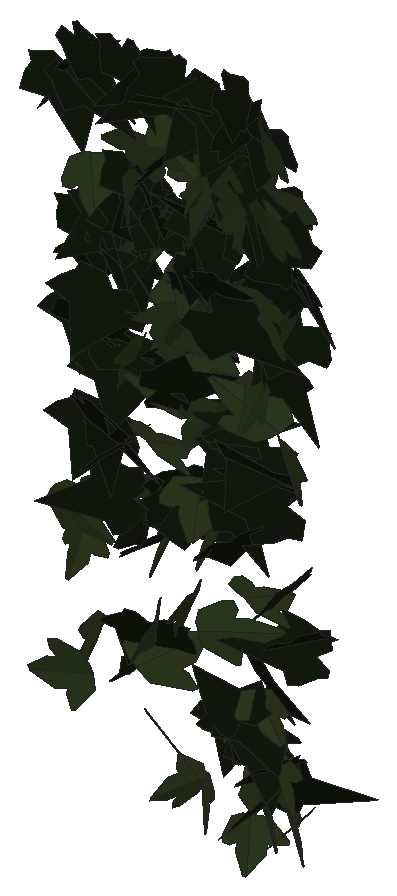
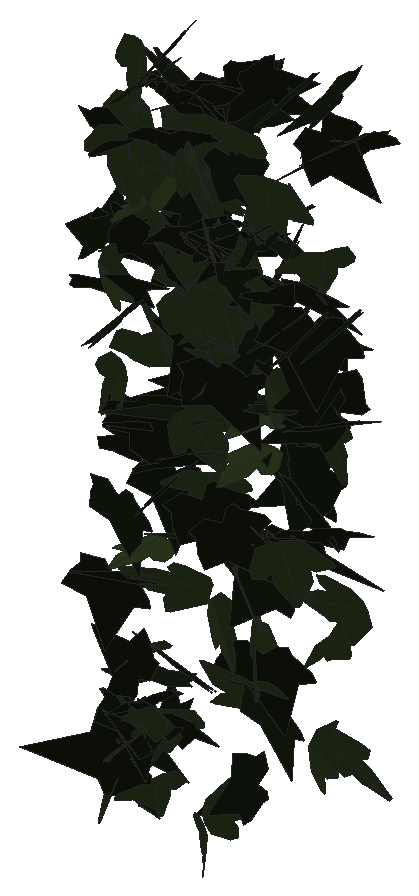
# SketchUp Ruby script. Lengths in inches.
U = 1.inch
M = Sketchup.active_model
def pt(a) = Geom::Point3d.new(a.map { |v| v * U })
def face(e, loops, mat)
  f = e.add_face(loops[0].map { |a| pt(a) })
  loops[1..].each { |l| e.add_face(l.map { |a| pt(a) }).erase! }
  f.material = f.back_material = mat if mat
  f
end
# faces: each face lists its corners as indices into pts; further lists are holes
def faces(e, pts, list, mat = nil) = list.each { |f| face(e, (f[0].is_a?(Array) ? f : [f]).map { |l| l.map { |i| pts[i] } }, mat) }
# xy, xz, yz: faces in a plane at the given z, y or x. An outline is a flat list of corners, or four numbers for a rectangle; further outlines are holes
def ring(l) = l.size == 4 ? [[l[0], l[1]], [l[2], l[1]], [l[2], l[3]], [l[0], l[3]]] : l.each_slice(2).to_a
def flat(e, list, mat, &to3) = list.each { |f| face(e, (f[0].is_a?(Array) ? f : [f]).map { |l| ring(l).map { |u, v| to3.(u, v) } }, mat) }
def xy(e, z, list, mat = nil) = flat(e, list, mat) { |x, y| [x, y, z] }
def xz(e, y, list, mat = nil) = flat(e, list, mat) { |x, z| [x, y, z] }
def yz(e, x, list, mat = nil) = flat(e, list, mat) { |y, z| [x, y, z] }
def lines(e, pts, list) = list.each { |a, b| e.add_line(pt(pts[a]), pt(pts[b])) }
# prism: a flat outline (further loops are holes) pulled along v
def prism(e, loops, v, mat = nil)
  f = face(e, loops, mat); d = Geom::Vector3d.new(v.map { |x| x * U })
  f.pushpull(f.normal.samedirection?(d) ? d.length : -d.length)
end
def box(e, o, s, mat = nil) = prism(e, [[o, [o[0] + s[0], o[1], o[2]], [o[0] + s[0], o[1] + s[1], o[2]], [o[0], o[1] + s[1], o[2]]]], [0, 0, s[2]], mat)
def at(x, y, z, deg = 0) = Geom::Transformation.translation(pt([x, y, z])) * Geom::Transformation.rotation(ORIGIN, Z_AXIS, deg.degrees)
def axes(o, x, y, z) = Geom::Transformation.new([*x, 0, *y, 0, *z, 0, *pt(o).to_a, 1])
def part(name) = M.definitions.add(name)
# library, detail: a bought-in or finely detailed component or shape, given as its bounding box
def library(name, o, s) = part(name).tap { |d| box(d.entities, o, s) }
def detail(e, o, s) = box(e.add_group.entities, o, s)
def put(e, d, t, mat = nil) = e.add_instance(d, t).tap { |i| i.material = mat if mat }
def group(e, t, mat = nil) = e.add_group.tap { |g| g.transformation = t; g.material = mat if mat }.entities
root = M.entities
M.materials.add("1026 AP 7946 SUNNY SIDE UP").color = [254, 231, 186]
M.materials.add("efeu1").color = [18, 25, 13]
M.materials.add("efeu2").color = [43, 57, 29]
c1 = part("ivyleaf_9")
p = [[1.54,2.16,1.25],[1.36,2.04,1.19],[-0.21,0.99,0.68],[-0.71,1.11,0.82],[-0.85,0.86,0.67],[-0.8,0.17,0.21],
  [-0.9,-0.01,0.1],[-0.67,-0.16,-0.02],[-0.08,-0.08,-0.05],[-0.03,-0.6,-0.4],[0.65,-0.88,-0.66],[0.83,-0.6,-0.49],
  [1.29,-0.42,-0.43],[1.8125,-0.07,-0.26],[1.21,0.44,0.15]]
faces(c1.entities,p,[[0,1,2,3,4,5,6,7,8,9,10,11,12,13,14]],"efeu1")
c2 = part("ivyleaf_10")
p = [[0,0.5,-0.03],[-0.0625,2.02,-0.43],[-0.19,2.01,-0.46],[-0.54,1.05,-0.29],[-0.52,0.625,-0.18],[-0.83,0.76,-0.28],
  [-1.16,0.64,-0.33],[-1.15,0.33,-0.24],[-0.77,-0.39,0.02],[-0.3,-0.51,0.16],[0.04,-0.48,0.23],[-0.02,2.01,-0.4375],
  [-0.06,2.01,-0.43],[0.04,-0.49,0.23],[0.67,-0.49,0.14],[1.38,0.36,-0.2],[1.375,0.51,-0.24],[0.81,0.65,-0.19],
  [0.62,0.59,-0.15],[0.6,1.09,-0.28],[0.5,1.23,-0.31]]
faces(c2.entities,p,[[0,1,2,3,4,5,6,7,8,9,10],[11,12,0,13,14,15,16,17,18,19,20]],"efeu2")
put(root,c1,axes([143.41,211.93,287.63],[0.08136,-0.09528,-0.35388],[0.40127,0.25153,-0.03085],[0.39018,-0.23882,0.10552]),"1026 AP 7946 SUNNY SIDE UP")
put(root,c1,axes([143.9,212.18,281.15],[-0.12123,-0.30196,0.00126],[0.33808,-0.05702,-0.22521],[0.3334,-0.05197,0.22884]),"1026 AP 7946 SUNNY SIDE UP")
put(root,c1,axes([141.3125,212.1875,287.15],[-0.42147,-0.22894,-0.01041],[0.03804,-0.01481,-0.36217],[0.35824,-0.26778,0.02621]),"1026 AP 7946 SUNNY SIDE UP")
put(root,c2,axes([144.01,212.08,286.56],[0.39463,-0.26002,0.00335],[-0.01071,-0.01314,-0.37209],[0.40878,0.25067,-0.01298]),"1026 AP 7946 SUNNY SIDE UP")
put(root,c2,axes([143.26,212.08,284.1],[0.25547,-0.29209,0.0202],[-0.00356,-0.02557,-0.34416],[0.46048,0.16185,-0.01387]),"1026 AP 7946 SUNNY SIDE UP")
put(root,c1,axes([144.28,212.14,280.25],[-0.32379,0.15465,-0.20783],[0.15623,-0.19117,-0.25547],[-0.3691,-0.21659,0.07419]),"1026 AP 7946 SUNNY SIDE UP")
put(root,c2,axes([144.35,211.98,289.41],[-0.49151,0.19025,0.03407],[-0.06783,-0.00956,-0.37572],[-0.29566,-0.31407,0.02956]),"1026 AP 7946 SUNNY SIDE UP")
put(root,c2,axes([140.92,211.97,281.06],[0.23147,-0.12831,-0.30768],[-0.41671,0.14112,-0.19667],[0.29416,0.30087,-0.0365]),"1026 AP 7946 SUNNY SIDE UP")
put(root,c1,axes([143.72,211.88,284.15],[0.1204,0.33371,-0.01462],[0.00758,-0.01761,-0.35271],[-0.52528,0.07624,-0.00844]),"1026 AP 7946 SUNNY SIDE UP")
put(root,c2,axes([143.72,211.93,289.44],[0.33583,-0.19793,-0.23762],[-0.16612,0.21457,-0.29063],[0.44668,0.2286,0.07057]),"1026 AP 7946 SUNNY SIDE UP")
put(root,c2,axes([143.39,211.95,282.6],[0.11849,-0.03815,-0.34108],[0.50138,0.10625,0.06281],[0.15127,-0.32228,0.05897]),"1026 AP 7946 SUNNY SIDE UP")
put(root,c2,axes([143.88,212.12,279.56],[0.24931,0.27277,-0.07663],[-0.03408,-0.07508,-0.32491],[-0.4439,0.15896,-0.01809]),"1026 AP 7946 SUNNY SIDE UP")
put(root,c1,axes([143.82,211.91,281.35],[-0.01917,0.20589,0.2712],[-0.32084,0.20275,-0.17268],[-0.41437,-0.16651,0.12116]),"1026 AP 7946 SUNNY SIDE UP")
put(root,c2,axes([143.83,212.14,287.89],[-0.39003,0.14142,-0.23722],[0.29057,-0.14078,-0.29394],[-0.3115,-0.30839,0.02284]),"1026 AP 7946 SUNNY SIDE UP")
put(root,c1,axes([141.06,212.08,285.23],[0.5517,-0.13341,0.00571],[-0.00858,-0.03202,-0.3855],[0.20983,0.34946,-0.03078]),"1026 AP 7946 SUNNY SIDE UP")
put(root,c2,axes([142.24,211.97,282.27],[0.03491,-0.31978,-0.2382],[-0.01932,0.2291,-0.32887],[0.61853,0.0252,0.00317]),"1026 AP 7946 SUNNY SIDE UP")
put(root,c1,axes([141.57,211.83,284.82],[0.10991,0.29394,0.19526],[0.00399,0.19117,-0.30799],[-0.54852,0.06029,0.03689]),"1026 AP 7946 SUNNY SIDE UP")
put(root,c1,axes([141.68,212.18,284],[-0.48126,0.06284,0.16932],[-0.26194,0.00045,-0.32047],[-0.08743,-0.34723,0.02813]),"1026 AP 7946 SUNNY SIDE UP")
put(root,c1,axes([140.53,212.24,290.4],[-0.11808,-0.34281,-0.09509],[0.05371,0.08494,-0.36072],[0.55486,-0.08118,0.01468]),"1026 AP 7946 SUNNY SIDE UP")
put(root,c1,axes([144.65,211.99,288.87],[-0.14149,0.13175,0.36499],[-0.42233,0.23288,-0.15847],[-0.41664,-0.28081,0.03669]),"1026 AP 7946 SUNNY SIDE UP")
put(root,c2,axes([141.77,212.02,289],[-0.15652,0.32454,0.09007],[-0.15146,0.05789,-0.34122],[-0.50555,-0.11782,0.07434]),"1026 AP 7946 SUNNY SIDE UP")
put(root,c2,axes([143.98,212.22,281.55],[-0.12187,-0.30105,0.03919],[0.34108,-0.08359,-0.21701],[0.33414,-0.02447,0.23581]),"1026 AP 7946 SUNNY SIDE UP")
put(root,c1,axes([142.99,212.01,287.99],[0.53721,0.08163,0.00496],[0.01953,-0.03336,-0.36023],[-0.12704,0.34004,-0.03441]),"1026 AP 7946 SUNNY SIDE UP")
put(root,c2,axes([144.2,212.26,280.54],[-0.31299,0.06184,-0.23488],[0.21436,-0.21391,-0.18336],[-0.30402,-0.21449,0.11253]),"1026 AP 7946 SUNNY SIDE UP")
put(root,c1,axes([140.78,212.15,290.99],[0.34204,-0.30774,-0.10674],[-0.0671,0.09442,-0.38719],[0.50527,0.22086,0.02084]),"1026 AP 7946 SUNNY SIDE UP")
put(root,c1,axes([142.16,211.95,283.84],[-0.17767,0.26919,0.19859],[-0.17678,0.15869,-0.29762],[-0.4882,-0.15543,0.0355]),"1026 AP 7946 SUNNY SIDE UP")
put(root,c1,axes([143.98,212.28,280.83],[-0.07872,-0.30552,-0.02321],[0.03448,0.01744,-0.31826],[0.48028,-0.05133,0.01904]),"1026 AP 7946 SUNNY SIDE UP")
put(root,c2,axes([142.93,212.4375,289.52],[0.03132,-0.13747,0.35864],[0.16857,-0.33273,-0.1433],[0.56506,0.10688,0.02287]),"1026 AP 7946 SUNNY SIDE UP")
put(root,c2,axes([142.59,212.42,279.71],[0.01538,-0.01101,0.34418],[0.02165,-0.334,-0.0137],[0.52527,0.01409,-0.00951]),"1026 AP 7946 SUNNY SIDE UP")
put(root,c2,axes([144.04,212.22,286.04],[0.22644,0.2463,0.22778],[-0.28558,-0.14101,0.28467],[0.43333,-0.22164,0.06858]),"1026 AP 7946 SUNNY SIDE UP")
put(root,c1,axes([144.6,212.22,279.8],[-0.25004,0.22113,-0.16999],[0.09533,-0.15926,-0.27887],[-0.42445,-0.16603,0.03751]),"1026 AP 7946 SUNNY SIDE UP")
put(root,c1,axes([141.52,212.3125,286.03],[-0.39178,-0.20278,-0.10898],[0.14862,0.04929,-0.32999],[0.32657,-0.2657,0.01944]),"1026 AP 7946 SUNNY SIDE UP")
put(root,c2,axes([142.87,212.22,284.51],[0.43622,0.1999,-0.03647],[-0.01942,-0.04514,-0.35124],[-0.31894,0.27615,-0.02851]),"1026 AP 7946 SUNNY SIDE UP")
put(root,c2,axes([142.45,212.24,287.22],[-0.2313,-0.30162,0.0603],[-0.01111,-0.06345,-0.3454],[0.48351,-0.14575,0.02091]),"1026 AP 7946 SUNNY SIDE UP")
put(root,c1,axes([144.28,212.33,284.72],[-0.19555,-0.181,-0.28824],[-0.3065,-0.20136,0.2231],[-0.42331,0.22941,-0.02838]),"1026 AP 7946 SUNNY SIDE UP")
put(root,c1,axes([144.57,212.01,283.54],[-0.0817,0.33048,0.07729],[-0.01959,0.07209,-0.34422],[-0.53187,-0.05342,0.00081]),"1026 AP 7946 SUNNY SIDE UP")
put(root,c2,axes([144.08,212.2,279.95],[-0.19113,0.27298,-0.06975],[0.03233,-0.06662,-0.30812],[-0.44166,-0.12301,0.00763]),"1026 AP 7946 SUNNY SIDE UP")
put(root,c1,axes([142.02,212.51,290.76],[-0.0977,-0.12448,-0.35389],[0.2013,-0.33307,0.09874],[-0.53698,-0.10221,0.10141]),"1026 AP 7946 SUNNY SIDE UP")
put(root,c1,axes([143.4375,212.46,280.61],[-0.09227,-0.1275,0.30467],[0.03598,-0.30222,-0.131],[0.50618,-0.00176,0.06485]),"1026 AP 7946 SUNNY SIDE UP")
put(root,c2,axes([142.71,212.1,286.98],[-0.03131,-0.31698,0.20739],[0.01477,0.20292,0.32837],[-0.59179,0.02184,-0.00278]),"1026 AP 7946 SUNNY SIDE UP")
put(root,c1,axes([142.02,212.17,282.11],[0.29024,0.18368,-0.22322],[-0.22101,-0.16693,-0.26881],[-0.38958,0.23154,-0.01381]),"1026 AP 7946 SUNNY SIDE UP")
put(root,c1,axes([142.34,212.49,290.76],[-0.0099,-0.02256,-0.41104],[0.00508,-0.39891,0.02085],[-0.62816,-0.00287,0.00664]),"1026 AP 7946 SUNNY SIDE UP")
put(root,c2,axes([143.0625,212.38,289.31],[-0.07957,-0.3237,0.16501],[0.02435,-0.16537,-0.33637],[0.56865,-0.03822,0.03749]),"1026 AP 7946 SUNNY SIDE UP")
put(root,c2,axes([140.4375,212.3125,283.49],[-0.21943,0.03722,-0.31921],[0.42465,-0.15615,-0.14544],[-0.24658,-0.30205,0.03359]),"1026 AP 7946 SUNNY SIDE UP")
put(root,c1,axes([142.35,212.52,290.42],[-0.5,-0.13518,0.07268],[0.18727,-0.32233,-0.08424],[0.15061,-0.04797,0.34602]),"1026 AP 7946 SUNNY SIDE UP")
put(root,c1,axes([144.01,212.41,284.93],[-0.50974,-0.04518,0.03072],[0.08466,-0.29057,0.14655],[0.01071,0.14686,0.30372]),"1026 AP 7946 SUNNY SIDE UP")
put(root,c1,axes([144.22,212.13,280.59],[0.05058,0.30453,-0.04296],[-0.00274,-0.04348,-0.31571],[-0.48368,0.03209,-0.00271]),"1026 AP 7946 SUNNY SIDE UP")
put(root,c2,axes([141.65,212.375,286.34],[0.08349,-0.32864,0.10656],[0.0434,-0.10215,-0.34338],[0.54089,0.05892,0.0111]),"1026 AP 7946 SUNNY SIDE UP")
put(root,c1,axes([143.88,212.47,285.42],[-0.39687,-0.24598,0.02536],[-0.0039,-0.03466,-0.3625],[0.38891,-0.25136,0.02225]),"1026 AP 7946 SUNNY SIDE UP")
put(root,c1,axes([144.74,212.41,282.46],[-0.36792,0.0572,0.23767],[-0.3667,-0.11574,-0.21508],[0.06962,-0.30729,0.12314]),"1026 AP 7946 SUNNY SIDE UP")
put(root,c2,axes([144.11,212.23,290.46],[-0.39882,0.26158,0.06328],[-0.13253,0.00064,-0.37035],[-0.40061,-0.26062,0.05953]),"1026 AP 7946 SUNNY SIDE UP")
put(root,c2,axes([140.67,212.43,283],[0.11876,0.25063,-0.21053],[-0.07072,-0.20115,-0.27057],[-0.50498,0.08711,-0.01162]),"1026 AP 7946 SUNNY SIDE UP")
put(root,c1,axes([142.32,212.06,286],[0.18885,0.09926,0.34778],[0.48539,0.14028,-0.15507],[-0.26382,0.32914,-0.03635]),"1026 AP 7946 SUNNY SIDE UP")
put(root,c1,axes([140.68,212.31,286.39],[0.5188,0.09944,-0.0951],[0.12409,0.0586,0.35379],[0.17429,-0.33772,0.03118]),"1026 AP 7946 SUNNY SIDE UP")
put(root,c1,axes([141.08,212.46,284.91],[-0.29597,-0.04534,-0.29409],[0.45382,-0.04136,-0.1897],[-0.01578,-0.33921,0.06038]),"1026 AP 7946 SUNNY SIDE UP")
put(root,c1,axes([143.61,212.28,290.53],[-0.39729,0.25709,0.00785],[-0.04407,-0.01894,-0.36987],[-0.40196,-0.25203,0.03279]),"1026 AP 7946 SUNNY SIDE UP")
put(root,c1,axes([141.35,212.45,290.88],[0.15703,-0.35013,-0.00324],[-0.01193,-0.00097,-0.37501],[0.55042,0.09987,-0.00721]),"1026 AP 7946 SUNNY SIDE UP")
put(root,c1,axes([143.28,212.37,284.48],[0.19337,-0.31352,-0.11016],[-0.06058,0.09784,-0.34637],[0.51643,0.12887,0.00062]),"1026 AP 7946 SUNNY SIDE UP")
put(root,c2,axes([144.35,212.33,285.61],[-0.34758,0.25886,-0.07208],[0.04394,-0.06985,-0.35024],[-0.41996,-0.22155,0.02301]),"1026 AP 7946 SUNNY SIDE UP")
put(root,c2,axes([142.17,212.11,285.09],[0.4503,-0.11038,-0.13743],[0.14194,0.31492,-0.06728],[0.23144,0.02161,0.30866]),"1026 AP 7946 SUNNY SIDE UP")
put(root,c2,axes([143.89,212.15,280.27],[0.01798,-0.13927,-0.29469],[0.27351,0.24153,-0.11289],[0.41755,-0.15222,0.08663]),"1026 AP 7946 SUNNY SIDE UP")
put(root,c2,axes([142.61,212.38,282.65],[0.07908,-0.35964,-0.00568],[-0.00816,0.00278,-0.37405],[0.56546,0.05033,-0.00461]),"1026 AP 7946 SUNNY SIDE UP")
put(root,c2,axes([142.02,212.22,281.53],[0.41449,-0.01938,-0.26172],[0.38676,0.11412,0.25474],[0.10381,-0.34777,0.09591]),"1026 AP 7946 SUNNY SIDE UP")
put(root,c1,axes([141.28,212.42,286.23],[0.15313,-0.32483,-0.03844],[0.32231,0.08956,-0.26458],[0.40014,0.05218,0.22783]),"1026 AP 7946 SUNNY SIDE UP")
put(root,c1,axes([142.65,212.26,288.1],[0.28053,-0.21406,-0.23159],[-0.21208,0.17852,-0.2859],[0.43808,0.2235,0.0099]),"1026 AP 7946 SUNNY SIDE UP")
put(root,c1,axes([143.03,212.56,288.6],[-0.54058,-0.01295,0.01761],[0.02503,-0.33813,0.06377],[0.02273,0.06449,0.34865]),"1026 AP 7946 SUNNY SIDE UP")
put(root,c2,axes([142.625,212.43,287.92],[0.25209,0.27898,-0.12192],[-0.09191,-0.10473,-0.33209],[-0.46855,0.17064,-0.00046]),"1026 AP 7946 SUNNY SIDE UP")
put(root,c1,axes([141.45,212.64,288.18],[-0.08028,-0.10277,0.3436],[-0.11027,-0.32779,-0.11682],[0.53848,-0.08245,0.0273]),"1026 AP 7946 SUNNY SIDE UP")
put(root,c1,axes([140.57,212.35,290.37],[0.22361,-0.28578,-0.17252],[0.01889,0.1849,-0.31655],[0.5192,0.11635,0.08582]),"1026 AP 7946 SUNNY SIDE UP")
put(root,c2,axes([143.92,212.38,289.17],[0.46289,-0.16695,-0.10596],[-0.13476,0.05543,-0.34827],[0.27645,0.30655,0.00765]),"1026 AP 7946 SUNNY SIDE UP")
put(root,c1,axes([143.0625,212.65,290.28],[-0.26571,-0.28353,0.13642],[0.03043,-0.16139,-0.32752],[0.49219,-0.14309,0.0939]),"1026 AP 7946 SUNNY SIDE UP")
put(root,c1,axes([142.93,212.59,290.55],[-0.46781,-0.20359,0.03358],[-0.00344,-0.05611,-0.36883],[0.32448,-0.29412,0.04451]),"1026 AP 7946 SUNNY SIDE UP")
put(root,c1,axes([143.35,212.27,290.99],[0.28593,-0.18597,-0.25311],[-0.20621,0.2101,-0.26374],[0.43698,0.22084,0.04116]),"1026 AP 7946 SUNNY SIDE UP")
put(root,c1,axes([141.76,212.64,286.94],[-0.02942,-0.13611,0.32228],[0.11653,-0.30823,-0.13506],[0.52478,0.06081,0.04806]),"1026 AP 7946 SUNNY SIDE UP")
put(root,c1,axes([141.79,212.25,288.61],[-0.18247,0.30542,0.12814],[-0.17574,0.08575,-0.32843],[-0.48677,-0.14545,0.07054]),"1026 AP 7946 SUNNY SIDE UP")
put(root,c1,axes([141.48,212.55,289],[0.02424,-0.35435,-0.01165],[0.03302,0.0102,-0.36467],[0.5564,0.01483,0.02215]),"1026 AP 7946 SUNNY SIDE UP")
put(root,c2,axes([142.56,212.24,286.92],[-0.18776,-0.15319,-0.31043],[0.34305,0.20798,-0.19735],[0.40441,-0.24755,0.02328]),"1026 AP 7946 SUNNY SIDE UP")
put(root,c2,axes([143.01,212.43,289.67],[-0.41315,0.21025,-0.10423],[0.08686,-0.09382,-0.34512],[-0.3573,-0.26593,0.03663]),"1026 AP 7946 SUNNY SIDE UP")
put(root,c2,axes([143.87,212.1875,283.17],[0.43706,-0.09854,-0.13227],[0.16361,0.304,-0.00658],[0.19402,-0.03437,0.30349]),"1026 AP 7946 SUNNY SIDE UP")
put(root,c1,axes([141.86,212.23,281.46],[-0.06389,0.31689,0.10129],[-0.05425,0.09267,-0.32784],[-0.51805,-0.04879,0.02184]),"1026 AP 7946 SUNNY SIDE UP")
put(root,c2,axes([140.85,212.33,286.12],[-0.40525,0.13666,0.21371],[-0.32098,0.05188,-0.2973],[-0.2208,-0.32626,0.03995]),"1026 AP 7946 SUNNY SIDE UP")
put(root,c1,axes([140.67,212.41,286.35],[0.48388,-0.13704,0.01351],[0.02143,-0.00354,-0.34705],[0.21553,0.30802,0.00418]),"1026 AP 7946 SUNNY SIDE UP")
put(root,c1,axes([141.95,212.17,283.39],[0.21652,0.26097,0.18008],[0.0674,0.17185,-0.30064],[-0.48797,0.13953,0.03838]),"1026 AP 7946 SUNNY SIDE UP")
put(root,c1,axes([142.23,212.35,283.9],[0.38509,-0.19923,-0.08659],[0.19173,0.23124,-0.20002],[0.27996,0.11569,0.25608]),"1026 AP 7946 SUNNY SIDE UP")
put(root,c1,axes([141.92,212.46,280.375],[0.44292,-0.20168,-0.00803],[-0.03119,-0.01631,-0.35608],[0.31576,0.28129,-0.0239]),"1026 AP 7946 SUNNY SIDE UP")
put(root,c1,axes([143.89,212.65,289.4375],[-0.22995,-0.32776,0.02342],[-0.001,-0.02664,-0.36975],[0.51682,-0.14588,0.00971]),"1026 AP 7946 SUNNY SIDE UP")
put(root,c2,axes([143.2,212.21,287.51],[0.05192,-0.13179,0.34019],[-0.08759,0.32639,0.14153],[-0.55326,-0.06404,0.00952]),"1026 AP 7946 SUNNY SIDE UP")
put(root,c2,axes([140.7,212.67,281.37],[0.09197,-0.25122,0.26622],[0.16514,-0.24006,-0.26485],[0.54379,0.11539,0.0354]),"1026 AP 7946 SUNNY SIDE UP")
put(root,c1,axes([140.69,212.5625,290.59],[-0.15966,0.2235,-0.27877],[0.12822,-0.26032,-0.25336],[-0.53834,-0.12829,0.02233]),"1026 AP 7946 SUNNY SIDE UP")
put(root,c1,axes([143.69,212.73,290.32],[-0.09889,-0.30338,0.18322],[0.00951,-0.18331,-0.31794],[0.55426,-0.05098,0.03815]),"1026 AP 7946 SUNNY SIDE UP")
put(root,c2,axes([142.08,212.54,283.42],[0.22255,-0.31363,0.03695],[0.00365,-0.04022,-0.35441],[0.49668,0.14082,-0.01395]),"1026 AP 7946 SUNNY SIDE UP")
put(root,c2,axes([141.93,212.22,285.84],[0.45412,-0.0825,-0.1606],[0.14352,0.32562,-0.00144],[0.23655,-0.03917,0.30918]),"1026 AP 7946 SUNNY SIDE UP")
put(root,c2,axes([141.4,212.52,284.02],[-0.37532,-0.22707,0.06926],[-0.04338,-0.06997,-0.3383],[0.37042,-0.23827,0.03056]),"1026 AP 7946 SUNNY SIDE UP")
put(root,c1,axes([141.23,212.63,288.15],[-0.53553,-0.06049,0.02293],[-0.02672,-0.03311,-0.35525],[0.09796,-0.33972,0.02847]),"1026 AP 7946 SUNNY SIDE UP")
put(root,c1,axes([141.68,212.74,288.63],[0.00866,-0.23684,0.26642],[0.07446,-0.25712,-0.24387],[0.54793,0.03868,0.02893]),"1026 AP 7946 SUNNY SIDE UP")
put(root,c2,axes([142.56,212.55,286.57],[0.50422,0.11506,-0.06847],[-0.0807,-0.05471,-0.34959],[-0.19328,0.32301,-0.03264]),"1026 AP 7946 SUNNY SIDE UP")
put(root,c1,axes([142.27,212.51,289.65],[-0.21816,0.29877,-0.18284],[0.08405,-0.17232,-0.33967],[-0.5413,-0.14717,0.02095]),"1026 AP 7946 SUNNY SIDE UP")
put(root,c1,axes([143.3125,212.63,281.01],[-0.4029,-0.12402,-0.14986],[0.24343,0.00613,-0.28766],[0.1749,-0.29423,0.05515]),"1026 AP 7946 SUNNY SIDE UP")
put(root,c1,axes([143.06,212.64,290.44],[-0.45873,-0.11618,-0.18777],[0.29567,0.01236,-0.31926],[0.16584,-0.34342,0.04979]),"1026 AP 7946 SUNNY SIDE UP")
put(root,c1,axes([144.41,212.34,282.5625],[0.17353,0.29793,-0.01607],[0.00567,-0.01977,-0.32726],[-0.46923,0.10994,-0.0099]),"1026 AP 7946 SUNNY SIDE UP")
put(root,c2,axes([142.7,212.51,286.74],[-0.46067,-0.20315,0.07761],[0.07504,0.06506,0.36671],[-0.33298,0.29572,-0.02473]),"1026 AP 7946 SUNNY SIDE UP")
put(root,c2,axes([142.36,212.53,290.03],[0.52315,0.12818,0.11737],[0.18601,0.00632,-0.3655],[-0.19418,0.35138,-0.03391]),"1026 AP 7946 SUNNY SIDE UP")
put(root,c1,axes([142,212.48,288.53],[0.04171,-0.25838,-0.2411],[0.03028,0.23398,-0.26416],[0.54577,0.00677,0.03308]),"1026 AP 7946 SUNNY SIDE UP")
put(root,c2,axes([143.3125,212.54,280.95],[0.38236,0.20691,-0.00279],[0.01923,-0.02035,-0.32816],[-0.32484,0.24235,-0.02271]),"1026 AP 7946 SUNNY SIDE UP")
put(root,c1,axes([144.04,212.61,286.6875],[0.19116,-0.32031,-0.03898],[-0.02277,0.03303,-0.35275],[0.50632,0.12242,-0.00115]),"1026 AP 7946 SUNNY SIDE UP")
put(root,c1,axes([143.71,212.72,281.49],[0.12537,-0.14144,0.30356],[0.20466,-0.26538,-0.16861],[0.47267,0.15242,-0.00751]),"1026 AP 7946 SUNNY SIDE UP")
put(root,c2,axes([142.03,212.67,288.44],[-0.00907,0.27062,-0.21556],[-0.12011,-0.20653,-0.27223],[-0.52583,0.04251,0.0659]),"1026 AP 7946 SUNNY SIDE UP")
put(root,c2,axes([142.8,212.65,285.57],[-0.25059,-0.26878,0.14076],[-0.08128,-0.12965,-0.32202],[0.46819,-0.16637,0.01944]),"1026 AP 7946 SUNNY SIDE UP")
put(root,c1,axes([140.54,212.76,286.375],[-0.2443,-0.29554,0.02533],[0.10134,-0.06256,-0.33276],[0.45539,-0.14462,0.08764]),"1026 AP 7946 SUNNY SIDE UP")
put(root,c1,axes([140.76,212.76,284.7],[-0.35745,-0.24773,0.01543],[0.06372,-0.05894,-0.33921],[0.38515,-0.22016,0.07044]),"1026 AP 7946 SUNNY SIDE UP")
put(root,c1,axes([143.1,212.73,289.83],[-0.35911,-0.25624,-0.08274],[0.13736,0.02682,-0.35024],[0.39856,-0.24012,0.04616]),"1026 AP 7946 SUNNY SIDE UP")
put(root,c2,axes([143.65,212.71,289.09],[-0.0828,-0.30449,0.16178],[-0.04658,-0.156,-0.31924],[0.53794,-0.06037,-0.00274]),"1026 AP 7946 SUNNY SIDE UP")
put(root,c2,axes([142.32,212.61,287.37],[0.34379,0.24892,-0.07739],[-0.06172,-0.06729,-0.34137],[-0.4048,0.22166,-0.01367]),"1026 AP 7946 SUNNY SIDE UP")
put(root,c2,axes([140.6875,212.59,288.76],[0.28556,0.30285,-0.03667],[-0.00037,-0.04329,-0.36334],[-0.47981,0.18028,-0.02154]),"1026 AP 7946 SUNNY SIDE UP")
put(root,c1,axes([142.71,212.36,286.8125],[0.31814,0.26519,0.07092],[0.08676,0.04248,-0.34289],[-0.42137,0.20896,-0.01705]),"1026 AP 7946 SUNNY SIDE UP")
put(root,c1,axes([142.25,212.68,284.24],[-0.04461,0.1866,-0.28769],[0.01581,-0.28071,-0.19519],[-0.52926,-0.02411,0.01842]),"1026 AP 7946 SUNNY SIDE UP")
put(root,c2,axes([142.875,212.7,287.37],[-0.34256,-0.16704,0.22089],[-0.20074,-0.18106,-0.27877],[0.37864,-0.24711,0.05206]),"1026 AP 7946 SUNNY SIDE UP")
put(root,c1,axes([142.62,212.65,284.45],[-0.01079,0.19729,-0.28404],[-0.11178,-0.2716,-0.19918],[-0.52271,0.05401,0.04846]),"1026 AP 7946 SUNNY SIDE UP")
put(root,c2,axes([142.55,212.63,288.54],[0.16374,-0.32643,-0.00403],[0.01593,0.0054,-0.35276],[0.51304,0.10401,0.01224]),"1026 AP 7946 SUNNY SIDE UP")
put(root,c1,axes([141.23,212.8,287.58],[0.01943,-0.3281,0.10699],[0.03047,-0.10496,-0.33852],[0.54117,0.01769,0.01522]),"1026 AP 7946 SUNNY SIDE UP")
put(root,c2,axes([142.73,212.66,289.42],[0.26767,-0.31407,-0.00034],[-0.02689,-0.01092,-0.36749],[0.49311,0.16989,-0.01985]),"1026 AP 7946 SUNNY SIDE UP")
put(root,c2,axes([143.52,212.46,288.82],[0.35164,-0.26087,-0.08992],[0.30732,0.22892,-0.19091],[0.30335,0.07048,0.29764]),"1026 AP 7946 SUNNY SIDE UP")
put(root,c2,axes([144.24,212.59,279.6],[-0.1954,0.28126,-0.03772],[0.0094,-0.03911,-0.31683],[-0.44622,-0.12399,0.00985]),"1026 AP 7946 SUNNY SIDE UP")
put(root,c2,axes([144.1,212.8,287.47],[0.15228,-0.26909,0.22096],[0.09825,-0.20697,-0.29568],[0.5336,0.1149,-0.00862]),"1026 AP 7946 SUNNY SIDE UP")
put(root,c1,axes([141.41,212.8,288.09],[-0.23921,-0.31264,-0.00296],[0.02444,-0.00635,-0.35781],[0.491,-0.152,0.01637]),"1026 AP 7946 SUNNY SIDE UP")
put(root,c2,axes([141.71,212.71,287.89],[-0.08238,-0.32514,0.10603],[-0.03828,-0.10217,-0.33979],[0.53577,-0.05729,-0.00798]),"1026 AP 7946 SUNNY SIDE UP")
put(root,c1,axes([142.4,212.6,286.47],[0.05205,0.27757,-0.21038],[-0.05751,-0.20275,-0.28899],[-0.54027,0.04833,0.0105]),"1026 AP 7946 SUNNY SIDE UP")
put(root,c1,axes([142.78,212.78,288.57],[-0.19602,-0.34028,-0.03737],[0.03358,0.02874,-0.37302],[0.53672,-0.12607,0.00969]),"1026 AP 7946 SUNNY SIDE UP")
put(root,c1,axes([144.1875,212.82,287.31],[-0.43707,-0.20335,0.02035],[0.01713,-0.04998,-0.35182],[0.32097,-0.27423,0.04649]),"1026 AP 7946 SUNNY SIDE UP")
put(root,c1,axes([143.15,212.88,284.96],[-0.31875,-0.24829,0.1351],[-0.04291,-0.14524,-0.32412],[0.44048,-0.19382,0.06619]),"1026 AP 7946 SUNNY SIDE UP")
put(root,c1,axes([143.02,212.4,285.53],[0.51544,-0.03783,-0.04192],[0.02845,0.30266,-0.13871],[0.08235,0.13225,0.31033]),"1026 AP 7946 SUNNY SIDE UP")
put(root,c2,axes([141.62,212.61,289.42],[-0.55974,-0.03535,0.01062],[-0.01139,-0.03294,-0.36724],[0.05686,-0.35461,0.03094]),"1026 AP 7946 SUNNY SIDE UP")
put(root,c1,axes([140.34,212.78,287.81],[0.12183,-0.33695,0.03111],[0.00068,-0.03284,-0.3563],[0.53222,0.07717,-0.00667]),"1026 AP 7946 SUNNY SIDE UP")
put(root,c2,axes([142.54,212.76,286.11],[0.10641,0.26412,-0.21128],[-0.13529,-0.19002,-0.28042],[-0.5096,0.1056,0.03033]),"1026 AP 7946 SUNNY SIDE UP")
put(root,c2,axes([143.95,212.625,289.37],[-0.54358,-0.02807,0.01807],[-0.02312,-0.03651,-0.35569],[0.04678,-0.34422,0.0342]),"1026 AP 7946 SUNNY SIDE UP")
put(root,c1,axes([140.875,212.54,287.64],[0.26592,0.28429,-0.13337],[-0.06681,-0.12676,-0.34044],[-0.48769,0.17238,-0.02608]),"1026 AP 7946 SUNNY SIDE UP")
put(root,c1,axes([142.75,212.79,288.44],[-0.51315,-0.06217,-0.08183],[0.13663,-0.03896,-0.33809],[0.0797,-0.33353,0.0527]),"1026 AP 7946 SUNNY SIDE UP")
put(root,c1,axes([142.09,212.82,288.29],[-0.3542,0.11008,-0.24781],[0.20042,-0.23253,-0.23335],[-0.36551,-0.23417,0.11219]),"1026 AP 7946 SUNNY SIDE UP")
put(root,c1,axes([143.96,212.5,280.0625],[0.30825,0.06655,0.31223],[0.47491,0.03932,-0.21019],[-0.10932,0.35848,-0.03271]),"1026 AP 7946 SUNNY SIDE UP")
put(root,c1,axes([144.09,212.65,288.17],[0.01201,-0.0412,-0.35179],[-0.51632,-0.10176,0.00449],[-0.15974,0.32581,-0.04096]),"1026 AP 7946 SUNNY SIDE UP")
put(root,c2,axes([142.55,212.77,279.49],[-0.21528,0.20866,-0.19723],[0.04338,-0.20307,-0.24799],[-0.44442,-0.12089,0.07133]),"1026 AP 7946 SUNNY SIDE UP")
put(root,c2,axes([142.56,212.72,289.3],[0.53557,-0.09393,0.04783],[0.07112,-0.01264,-0.36406],[0.14903,0.34359,0.00184]),"1026 AP 7946 SUNNY SIDE UP")
put(root,c1,axes([140.83,212.86,287.6],[0.08273,-0.32537,0.0985],[0.00044,-0.09858,-0.33978],[0.53408,0.05048,-0.01498]),"1026 AP 7946 SUNNY SIDE UP")
put(root,c1,axes([144.11,212.83,288.12],[0.23101,-0.28954,0.12531],[0.0614,-0.11823,-0.33469],[0.491,0.15101,-0.01711]),"1026 AP 7946 SUNNY SIDE UP")
